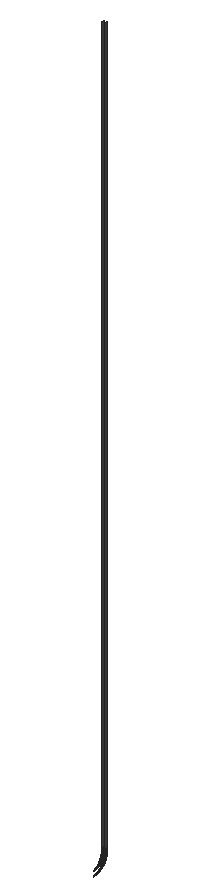
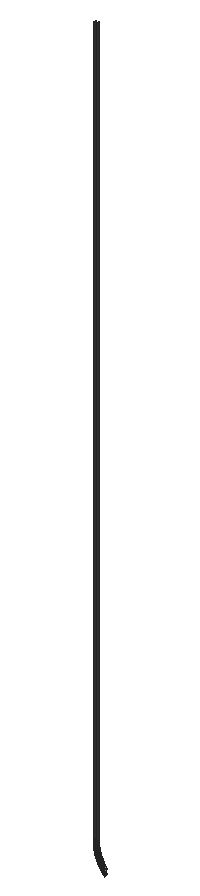
# SketchUp Ruby script. Lengths in inches.
U = 1.inch
M = Sketchup.active_model
def pt(a) = Geom::Point3d.new(a.map { |v| v * U })
def face(e, loops, mat)
  f = e.add_face(loops[0].map { |a| pt(a) })
  loops[1..].each { |l| e.add_face(l.map { |a| pt(a) }).erase! }
  f.material = f.back_material = mat if mat
  f
end
# faces: each face lists its corners as indices into pts; further lists are holes
def faces(e, pts, list, mat = nil) = list.each { |f| face(e, (f[0].is_a?(Array) ? f : [f]).map { |l| l.map { |i| pts[i] } }, mat) }
# xy, xz, yz: faces in a plane at the given z, y or x. An outline is a flat list of corners, or four numbers for a rectangle; further outlines are holes
def ring(l) = l.size == 4 ? [[l[0], l[1]], [l[2], l[1]], [l[2], l[3]], [l[0], l[3]]] : l.each_slice(2).to_a
def flat(e, list, mat, &to3) = list.each { |f| face(e, (f[0].is_a?(Array) ? f : [f]).map { |l| ring(l).map { |u, v| to3.(u, v) } }, mat) }
def xy(e, z, list, mat = nil) = flat(e, list, mat) { |x, y| [x, y, z] }
def xz(e, y, list, mat = nil) = flat(e, list, mat) { |x, z| [x, y, z] }
def yz(e, x, list, mat = nil) = flat(e, list, mat) { |y, z| [x, y, z] }
def lines(e, pts, list) = list.each { |a, b| e.add_line(pt(pts[a]), pt(pts[b])) }
# prism: a flat outline (further loops are holes) pulled along v
def prism(e, loops, v, mat = nil)
  f = face(e, loops, mat); d = Geom::Vector3d.new(v.map { |x| x * U })
  f.pushpull(f.normal.samedirection?(d) ? d.length : -d.length)
end
def box(e, o, s, mat = nil) = prism(e, [[o, [o[0] + s[0], o[1], o[2]], [o[0] + s[0], o[1] + s[1], o[2]], [o[0], o[1] + s[1], o[2]]]], [0, 0, s[2]], mat)
def at(x, y, z, deg = 0) = Geom::Transformation.translation(pt([x, y, z])) * Geom::Transformation.rotation(ORIGIN, Z_AXIS, deg.degrees)
def axes(o, x, y, z) = Geom::Transformation.new([*x, 0, *y, 0, *z, 0, *pt(o).to_a, 1])
def part(name) = M.definitions.add(name)
# library, detail: a bought-in or finely detailed component or shape, given as its bounding box
def library(name, o, s) = part(name).tap { |d| box(d.entities, o, s) }
def detail(e, o, s) = box(e.add_group.entities, o, s)
def put(e, d, t, mat = nil) = e.add_instance(d, t).tap { |i| i.material = mat if mat }
def group(e, t, mat = nil) = e.add_group.tap { |g| g.transformation = t; g.material = mat if mat }.entities
root = M.entities
M.materials.add("1432 AP 8245 TAR ROAD").color = [71, 72, 75]
M.materials.add("Outer Light").color = [251, 217, 152]
yz(root,555.99,[[95.37,191.05,96.87,191.2],[95.37,191.2,96.87,191.34]],"1432 AP 8245 TAR ROAD")
yz(root,555.99,[[95.37,191.05,96.87,191.2],[95.37,191.2,96.87,191.34]],"Outer Light")
yz(root,556,[[95.37,191.49,96.87,191.64],[95.37,191.64,96.87,191.79],[95.37,191.79,96.87,560.79]],"1432 AP 8245 TAR ROAD")
yz(root,556,[[95.37,191.49,96.87,191.64],[95.37,191.64,96.87,191.79],[95.37,191.79,96.87,560.79]],"Outer Light")
yz(root,557.48,[[95.37,190.83,96.87,190.99]],"1432 AP 8245 TAR ROAD")
yz(root,557.48,[[95.37,190.83,96.87,190.99]],"Outer Light")
yz(root,557.49,[[95.37,191.15,96.87,191.31]],"1432 AP 8245 TAR ROAD")
yz(root,557.49,[[95.37,191.15,96.87,191.31]],"Outer Light")
yz(root,557.5,[[95.37,191.47,96.87,191.63],[95.37,191.63,96.87,191.79],[95.37,191.79,96.87,560.79]],"1432 AP 8245 TAR ROAD")
yz(root,557.5,[[95.37,191.47,96.87,191.63],[95.37,191.63,96.87,191.79],[95.37,191.79,96.87,560.79]],"Outer Light")
p = [[551.83,95.37,177.64],[551.94,95.37,177.76],[551.94,96.87,177.76],[551.83,96.87,177.64],[551.83,96.87,177.64],[551.94,96.87,177.76],
  [551.94,95.37,177.76],[551.83,95.37,177.64],[552.05,95.37,177.875],[552.05,96.87,177.875],[552.05,96.87,177.875],[552.05,95.37,177.875],
  [552.16,95.37,178],[552.16,96.87,178],[552.16,96.87,178],[552.16,95.37,178],[552.27,95.37,178.11],[552.27,96.87,178.11],
  [552.27,96.87,178.11],[552.27,95.37,178.11],[552.38,95.37,178.24],[552.38,96.87,178.24],[552.38,96.87,178.24],[552.38,95.37,178.24],
  [552.48,95.37,178.36],[552.48,96.87,178.36],[552.48,96.87,178.36],[552.48,95.37,178.36],[552.59,95.37,178.48],[552.59,96.87,178.48],
  [552.59,96.87,178.48],[552.59,95.37,178.48],[552.69,95.37,178.6],[552.69,96.87,178.6],[552.69,96.87,178.6],[552.69,95.37,178.6],
  [552.8,95.37,178.72],[552.8,96.87,178.72],[552.8,96.87,178.72],[552.8,95.37,178.72],[552.9,95.37,178.85],[552.9,96.87,178.85],
  [552.9,96.87,178.85],[552.9,95.37,178.85],[553,95.37,178.97],[553,96.87,178.97],[553,96.87,178.97],[553,95.37,178.97],
  [553.1,95.37,179.1],[553.1,96.87,179.1],[553.1,96.87,179.1],[553.1,95.37,179.1],[553.2,95.37,179.23],[553.2,96.87,179.23],
  [553.2,96.87,179.23],[553.2,95.37,179.23],[553.3,95.37,179.36],[553.3,96.87,179.36],[553.3,96.87,179.36],[553.3,95.37,179.36],
  [553.39,95.37,179.48],[553.39,96.87,179.48],[553.39,96.87,179.48],[553.39,95.37,179.48],[553.49,95.37,179.61],[553.49,96.87,179.61],
  [553.49,96.87,179.61],[553.49,95.37,179.61],[553.58,95.37,179.74],[553.58,96.87,179.74],[553.58,96.87,179.74],[553.58,95.37,179.74],
  [553.68,95.37,179.875],[553.68,96.87,179.875],[553.68,96.87,179.875],[553.68,95.37,179.875],[551.92,95.37,180.03],[551.83,95.37,179.91],
  [551.83,96.87,179.91],[551.92,96.87,180.03],[551.92,96.87,180.03],[551.83,96.87,179.91],[551.83,95.37,179.91],[551.92,95.37,180.03],
  [553.77,95.37,180],[553.77,96.87,180],[553.77,96.87,180],[553.77,95.37,180],[552.01,95.37,180.15],[552.01,96.87,180.15],
  [552.01,96.87,180.15],[552.01,95.37,180.15],[553.86,95.37,180.14],[553.86,96.87,180.14],[553.86,96.87,180.14],[553.86,95.37,180.14],
  [552.1,95.37,180.27],[552.1,96.87,180.27],[552.1,96.87,180.27],[552.1,95.37,180.27],[553.96,95.37,180.27],[553.96,96.87,180.27],
  [553.96,96.87,180.27],[553.96,95.37,180.27],[552.19,95.37,180.38],[552.19,96.87,180.38],[552.19,96.87,180.38],[552.19,95.37,180.38],
  [554.05,95.37,180.4],[554.05,96.87,180.4],[554.05,96.87,180.4],[554.05,95.37,180.4],[552.28,95.37,180.5],[552.28,96.87,180.5],
  [552.28,96.87,180.5],[552.28,95.37,180.5],[554.13,95.37,180.54],[554.13,96.87,180.54],[554.13,96.87,180.54],[554.13,95.37,180.54],
  [552.37,95.37,180.625],[552.37,96.87,180.625],[552.37,96.87,180.625],[552.37,95.37,180.625],[554.22,95.37,180.67],[554.22,96.87,180.67],
  [554.22,96.87,180.67],[554.22,95.37,180.67],[552.46,95.37,180.75],[552.46,96.87,180.75],[552.46,96.87,180.75],[552.46,95.37,180.75],
  [552.54,95.37,180.87],[552.54,96.87,180.87],[552.54,96.87,180.87],[552.54,95.37,180.87],[554.31,95.37,180.81],[554.31,96.87,180.81],
  [554.31,96.87,180.81],[554.31,95.37,180.81],[554.39,95.37,180.94],[554.39,96.87,180.94],[554.39,96.87,180.94],[554.39,95.37,180.94],
  [552.63,95.37,180.99],[552.63,96.87,180.99],[552.63,96.87,180.99],[552.63,95.37,180.99],[554.48,95.37,181.08],[554.48,96.87,181.08],
  [554.48,96.87,181.08],[554.48,95.37,181.08],[552.71,95.37,181.11],[552.71,96.87,181.11],[552.71,96.87,181.11],[552.71,95.37,181.11],
  [552.8,95.37,181.24],[552.8,96.87,181.24],[552.8,96.87,181.24],[552.8,95.37,181.24],[554.5625,95.37,181.22],[554.5625,96.87,181.22],
  [554.5625,96.87,181.22],[554.5625,95.37,181.22],[552.88,95.37,181.36],[552.88,96.87,181.36],[552.88,96.87,181.36],[552.88,95.37,181.36],
  [554.65,95.37,181.36],[554.65,96.87,181.36],[554.65,96.87,181.36],[554.65,95.37,181.36],[552.96,95.37,181.49],[552.96,96.87,181.49],
  [552.96,96.87,181.49],[552.96,95.37,181.49],[554.73,95.37,181.5],[554.73,96.87,181.5],[554.73,96.87,181.5],[554.73,95.37,181.5],
  [553.04,95.37,181.61],[553.04,96.87,181.61],[553.04,96.87,181.61],[553.04,95.37,181.61],[554.81,95.37,181.64],[554.81,96.87,181.64],
  [554.81,96.87,181.64],[554.81,95.37,181.64],[553.12,95.37,181.74],[553.12,96.87,181.74],[553.12,96.87,181.74],[553.12,95.37,181.74],
  [554.89,95.37,181.78],[554.89,96.87,181.78],[554.89,96.87,181.78],[554.89,95.37,181.78],[553.2,95.37,181.86],[553.2,96.87,181.86],
  [553.2,96.87,181.86],[553.2,95.37,181.86],[554.96,95.37,181.92],[554.96,96.87,181.92],[554.96,96.87,181.92],[554.96,95.37,181.92],
  [553.28,95.37,181.99],[553.28,96.87,181.99],[553.28,96.87,181.99],[553.28,95.37,181.99],[555.04,95.37,182.06],[555.04,96.87,182.06],
  [555.04,96.87,182.06],[555.04,95.37,182.06],[553.35,95.37,182.12],[553.35,96.87,182.12],[553.35,96.87,182.12],[553.35,95.37,182.12],
  [553.43,95.37,182.25],[553.43,96.87,182.25],[553.43,96.87,182.25],[553.43,95.37,182.25],[555.12,95.37,182.2],[555.12,96.87,182.2],
  [555.12,96.87,182.2],[555.12,95.37,182.2],[553.5,95.37,182.38],[553.5,96.87,182.38],[553.5,96.87,182.38],[553.5,95.37,182.38],
  [555.19,95.37,182.34],[555.19,96.87,182.34],[555.19,96.87,182.34],[555.19,95.37,182.34],[555.27,95.37,182.49],[555.27,96.87,182.49],
  [555.27,96.87,182.49],[555.27,95.37,182.49],[553.58,95.37,182.51],[553.58,96.87,182.51],[553.58,96.87,182.51],[553.58,95.37,182.51],
  [553.65,95.37,182.64],[553.65,96.87,182.64],[553.65,96.87,182.64],[553.65,95.37,182.64],[555.34,95.37,182.63],[555.34,96.87,182.63],
  [555.34,96.87,182.63],[555.34,95.37,182.63],[553.72,95.37,182.77],[553.72,96.87,182.77],[553.72,96.87,182.77],[553.72,95.37,182.77],
  [555.41,95.37,182.77],[555.41,96.87,182.77],[555.41,96.87,182.77],[555.41,95.37,182.77],[553.79,95.37,182.9],[553.79,96.87,182.9],
  [553.79,96.87,182.9],[553.79,95.37,182.9],[555.48,95.37,182.92],[555.48,96.87,182.92],[555.48,96.87,182.92],[555.48,95.37,182.92],
  [553.86,95.37,183.03],[553.86,96.87,183.03],[553.86,96.87,183.03],[553.86,95.37,183.03],[555.55,95.37,183.0625],[555.55,96.87,183.0625],
  [555.55,96.87,183.0625],[555.55,95.37,183.0625],[553.93,95.37,183.17],[553.93,96.87,183.17],[553.93,96.87,183.17],[553.93,95.37,183.17],
  [555.62,95.37,183.21],[555.62,96.87,183.21],[555.62,96.87,183.21],[555.62,95.37,183.21],[554,95.37,183.3],[554,96.87,183.3],
  [554,96.87,183.3],[554,95.37,183.3],[555.68,95.37,183.36],[555.68,96.87,183.36],[555.68,96.87,183.36],[555.68,95.37,183.36],
  [554.0625,95.37,183.43],[554.0625,96.87,183.43],[554.0625,96.87,183.43],[554.0625,95.37,183.43],[554.13,95.37,183.57],[554.13,96.87,183.57],
  [554.13,96.87,183.57],[554.13,95.37,183.57],[555.75,95.37,183.5],[555.75,96.87,183.5],[555.75,96.87,183.5],[555.75,95.37,183.5],
  [555.8125,95.37,183.65],[555.8125,96.87,183.65],[555.8125,96.87,183.65],[555.8125,95.37,183.65],[554.19,95.37,183.7],[554.19,96.87,183.7],
  [554.19,96.87,183.7],[554.19,95.37,183.7],[554.25,95.37,183.84],[554.25,96.87,183.84],[554.25,96.87,183.84],[554.25,95.37,183.84],
  [555.88,95.37,183.8],[555.88,96.87,183.8],[555.88,96.87,183.8],[555.88,95.37,183.8],[554.32,95.37,183.97],[554.32,96.87,183.97],
  [554.32,96.87,183.97],[554.32,95.37,183.97],[555.94,95.37,183.95],[555.94,96.87,183.95],[555.94,96.87,183.95],[555.94,95.37,183.95],
  [556,95.37,184.1],[556,96.87,184.1],[556,96.87,184.1],[556,95.37,184.1],[554.38,95.37,184.11],[554.38,96.87,184.11],
  [554.38,96.87,184.11],[554.38,95.37,184.11],[554.4375,95.37,184.25],[554.4375,96.87,184.25],[554.4375,96.87,184.25],[554.4375,95.37,184.25],
  [556.06,95.37,184.25],[556.06,96.87,184.25],[556.06,96.87,184.25],[556.06,95.37,184.25],[554.5,95.37,184.38],[554.5,96.87,184.38],
  [554.5,96.87,184.38],[554.5,95.37,184.38],[556.12,95.37,184.4],[556.12,96.87,184.4],[556.12,96.87,184.4],[556.12,95.37,184.4],
  [554.55,95.37,184.52],[554.55,96.87,184.52],[554.55,96.87,184.52],[554.55,95.37,184.52],[556.18,95.37,184.55],[556.18,96.87,184.55],
  [556.18,96.87,184.55],[556.18,95.37,184.55],[554.61,95.37,184.66],[554.61,96.87,184.66],[554.61,96.87,184.66],[554.61,95.37,184.66],
  [556.23,95.37,184.7],[556.23,96.87,184.7],[556.23,96.87,184.7],[556.23,95.37,184.7],[554.67,95.37,184.8],[554.67,96.87,184.8],
  [554.67,96.87,184.8],[554.67,95.37,184.8],[556.29,95.37,184.85],[556.29,96.87,184.85],[556.29,96.87,184.85],[556.29,95.37,184.85],
  [554.72,95.37,184.9375],[554.72,96.87,184.9375],[554.72,96.87,184.9375],[554.72,95.37,184.9375],[556.34,95.37,185],[556.34,96.87,185],
  [556.34,96.87,185],[556.34,95.37,185],[554.77,95.37,185.08],[554.77,96.87,185.08],[554.77,96.87,185.08],[554.77,95.37,185.08],
  [556.39,95.37,185.15],[556.39,96.87,185.15],[556.39,96.87,185.15],[556.39,95.37,185.15],[554.83,95.37,185.22],[554.83,96.87,185.22],
  [554.83,96.87,185.22],[554.83,95.37,185.22],[554.875,95.37,185.36],[554.875,96.87,185.36],[554.875,96.87,185.36],[554.875,95.37,185.36],
  [556.45,95.37,185.3],[556.45,96.87,185.3],[556.45,96.87,185.3],[556.45,95.37,185.3],[556.5,95.37,185.46],[556.5,96.87,185.46],
  [556.5,96.87,185.46],[556.5,95.37,185.46],[554.93,95.37,185.5],[554.93,96.87,185.5],[554.93,96.87,185.5],[554.93,95.37,185.5],
  [554.98,95.37,185.64],[554.98,96.87,185.64],[554.98,96.87,185.64],[554.98,95.37,185.64],[556.55,95.37,185.61],[556.55,96.87,185.61],
  [556.55,96.87,185.61],[556.55,95.37,185.61],[555.02,95.37,185.78],[555.02,96.87,185.78],[555.02,96.87,185.78],[555.02,95.37,185.78],
  [556.59,95.37,185.76],[556.59,96.87,185.76],[556.59,96.87,185.76],[556.59,95.37,185.76],[555.07,95.37,185.92],[555.07,96.87,185.92],
  [555.07,96.87,185.92],[555.07,95.37,185.92],[556.64,95.37,185.92],[556.64,96.87,185.92],[556.64,96.87,185.92],[556.64,95.37,185.92],
  [555.12,95.37,186.0625],[555.12,96.87,186.0625],[555.12,96.87,186.0625],[555.12,95.37,186.0625],[556.6875,95.37,186.07],[556.6875,96.87,186.07],
  [556.6875,96.87,186.07],[556.6875,95.37,186.07],[555.16,95.37,186.21],[555.16,96.87,186.21],[555.16,96.87,186.21],[555.16,95.37,186.21],
  [556.73,95.37,186.23],[556.73,96.87,186.23],[556.73,96.87,186.23],[556.73,95.37,186.23],[555.2,95.37,186.35],[555.2,96.87,186.35],
  [555.2,96.87,186.35],[555.2,95.37,186.35],[556.77,95.37,186.38],[556.77,96.87,186.38],[556.77,96.87,186.38],[556.77,95.37,186.38],
  [555.25,95.37,186.49],[555.25,96.87,186.49],[555.25,96.87,186.49],[555.25,95.37,186.49],[556.82,95.37,186.54],[556.82,96.87,186.54],
  [556.82,96.87,186.54],[556.82,95.37,186.54],[555.29,95.37,186.63],[555.29,96.87,186.63],[555.29,96.87,186.63],[555.29,95.37,186.63],
  [556.86,95.37,186.69],[556.86,96.87,186.69],[556.86,96.87,186.69],[556.86,95.37,186.69],[555.33,95.37,186.78],[555.33,96.87,186.78],
  [555.33,96.87,186.78],[555.33,95.37,186.78],[556.9,95.37,186.85],[556.9,96.87,186.85],[556.9,96.87,186.85],[556.9,95.37,186.85],
  [555.37,95.37,186.92],[555.37,96.87,186.92],[555.37,96.87,186.92],[555.37,95.37,186.92],[555.4,95.37,187.07],[555.4,96.87,187.07],
  [555.4,96.87,187.07],[555.4,95.37,187.07],[556.93,95.37,187.01],[556.93,96.87,187.01],[556.93,96.87,187.01],[556.93,95.37,187.01],
  [556.97,95.37,187.16],[556.97,96.87,187.16],[556.97,96.87,187.16],[556.97,95.37,187.16],[555.44,95.37,187.21],[555.44,96.87,187.21],
  [555.44,96.87,187.21],[555.44,95.37,187.21],[555.48,95.37,187.36],[555.48,96.87,187.36],[555.48,96.87,187.36],[555.48,95.37,187.36],
  [557.01,95.37,187.32],[557.01,96.87,187.32],[557.01,96.87,187.32],[557.01,95.37,187.32],[557.04,95.37,187.48],[557.04,96.87,187.48],
  [557.04,96.87,187.48],[557.04,95.37,187.48],[555.51,95.37,187.5],[555.51,96.87,187.5],[555.51,96.87,187.5],[555.51,95.37,187.5],
  [555.54,95.37,187.65],[555.54,96.87,187.65],[555.54,96.87,187.65],[555.54,95.37,187.65],[557.07,95.37,187.63],[557.07,96.87,187.63],
  [557.07,96.87,187.63],[557.07,95.37,187.63],[555.57,95.37,187.79],[555.57,96.87,187.79],[555.57,96.87,187.79],[555.57,95.37,187.79],
  [557.11,95.37,187.79],[557.11,96.87,187.79],[557.11,96.87,187.79],[557.11,95.37,187.79],[555.61,95.37,187.9375],[555.61,96.87,187.9375],
  [555.61,96.87,187.9375],[555.61,95.37,187.9375],[557.14,95.37,187.95],[557.14,96.87,187.95],[557.14,96.87,187.95],[557.14,95.37,187.95],
  [555.63,95.37,188.09],[555.63,96.87,188.09],[555.63,96.87,188.09],[555.63,95.37,188.09],[557.17,95.37,188.11],[557.17,96.87,188.11],
  [557.17,96.87,188.11],[557.17,95.37,188.11],[555.66,95.37,188.23],[555.66,96.87,188.23],[555.66,96.87,188.23],[555.66,95.37,188.23],
  [557.19,95.37,188.27],[557.19,96.87,188.27],[557.19,96.87,188.27],[557.19,95.37,188.27],[555.69,95.37,188.38],[555.69,96.87,188.38],
  [555.69,96.87,188.38],[555.69,95.37,188.38],[557.22,95.37,188.43],[557.22,96.87,188.43],[557.22,96.87,188.43],[557.22,95.37,188.43],
  [555.72,95.37,188.53],[555.72,96.87,188.53],[555.72,96.87,188.53],[555.72,95.37,188.53],[557.25,95.37,188.59],[557.25,96.87,188.59],
  [557.25,96.87,188.59],[557.25,95.37,188.59],[555.74,95.37,188.67],[555.74,96.87,188.67],[555.74,96.87,188.67],[555.74,95.37,188.67],
  [557.27,95.37,188.74],[557.27,96.87,188.74],[557.27,96.87,188.74],[557.27,95.37,188.74],[555.77,95.37,188.82],[555.77,96.87,188.82],
  [555.77,96.87,188.82],[555.77,95.37,188.82],[557.3,95.37,188.9],[557.3,96.87,188.9],[557.3,96.87,188.9],[557.3,95.37,188.9],
  [555.79,95.37,188.97],[555.79,96.87,188.97],[555.79,96.87,188.97],[555.79,95.37,188.97],[557.32,95.37,189.0625],[557.32,96.87,189.0625],
  [557.32,96.87,189.0625],[557.32,95.37,189.0625],[555.81,95.37,189.11],[555.81,96.87,189.11],[555.81,96.87,189.11],[555.81,95.37,189.11],
  [555.83,95.37,189.26],[555.83,96.87,189.26],[555.83,96.87,189.26],[555.83,95.37,189.26],[557.34,95.37,189.22],[557.34,96.87,189.22],
  [557.34,96.87,189.22],[557.34,95.37,189.22],[557.36,95.37,189.38],[557.36,96.87,189.38],[557.36,96.87,189.38],[557.36,95.37,189.38],
  [555.85,95.37,189.41],[555.85,96.87,189.41],[555.85,96.87,189.41],[555.85,95.37,189.41],[555.87,95.37,189.56],[555.87,96.87,189.56],
  [555.87,96.87,189.56],[555.87,95.37,189.56],[557.375,95.37,189.54],[557.375,96.87,189.54],[557.375,96.87,189.54],[557.375,95.37,189.54],
  [557.39,95.37,189.7],[557.39,96.87,189.7],[557.39,96.87,189.7],[557.39,95.37,189.7],[555.89,95.37,189.71],[555.89,96.87,189.71],
  [555.89,96.87,189.71],[555.89,95.37,189.71],[555.9,95.37,189.86],[555.9,96.87,189.86],[555.9,96.87,189.86],[555.9,95.37,189.86],
  [557.41,95.37,189.86],[557.41,96.87,189.86],[557.41,96.87,189.86],[557.41,95.37,189.86],[555.92,95.37,190],[555.92,96.87,190],
  [555.92,96.87,190],[555.92,95.37,190],[557.42,95.37,190.02],[557.42,96.87,190.02],[557.42,96.87,190.02],[557.42,95.37,190.02],
  [555.93,95.37,190.15],[555.93,96.87,190.15],[555.93,96.87,190.15],[555.93,95.37,190.15],[557.4375,95.37,190.18],[557.4375,96.87,190.18],
  [557.4375,96.87,190.18],[557.4375,95.37,190.18],[555.94,95.37,190.3],[555.94,96.87,190.3],[555.94,96.87,190.3],[555.94,95.37,190.3],
  [557.45,95.37,190.34],[557.45,96.87,190.34],[557.45,96.87,190.34],[557.45,95.37,190.34],[555.95,95.37,190.45],[555.95,96.87,190.45],
  [555.95,96.87,190.45],[555.95,95.37,190.45],[557.46,95.37,190.5],[557.46,96.87,190.5],[557.46,96.87,190.5],[557.46,95.37,190.5],
  [555.96,95.37,190.6],[555.96,96.87,190.6],[555.96,96.87,190.6],[555.96,95.37,190.6],[557.47,95.37,190.67],[557.47,96.87,190.67],
  [557.47,96.87,190.67],[557.47,95.37,190.67],[555.97,95.37,190.75],[555.97,96.87,190.75],[555.97,96.87,190.75],[555.97,95.37,190.75],
  [555.98,95.37,190.9],[555.98,96.87,190.9],[555.98,96.87,190.9],[555.98,95.37,190.9],[557.48,95.37,190.83],[557.48,96.87,190.83],
  [557.48,96.87,190.83],[557.48,95.37,190.83],[555.99,95.37,191.05],[555.99,96.87,191.05],[555.99,96.87,191.05],[555.99,95.37,191.05],
  [557.48,95.37,190.99],[557.49,95.37,191.15],[557.49,96.87,191.15],[557.48,96.87,190.99],[557.48,96.87,190.99],[557.49,96.87,191.15],
  [557.49,95.37,191.15],[557.48,95.37,190.99],[556,95.37,191.49],[555.99,95.37,191.34],[555.99,96.87,191.34],[556,96.87,191.49],
  [556,96.87,191.49],[555.99,96.87,191.34],[555.99,95.37,191.34],[556,95.37,191.49],[557.49,95.37,191.31],[557.5,95.37,191.47],
  [557.5,96.87,191.47],[557.49,96.87,191.31],[557.49,96.87,191.31],[557.5,96.87,191.47],[557.5,95.37,191.47],[557.49,95.37,191.31]]
faces(root,p,[[0,1,2,3],[1,8,9,2],[8,12,13,9],[12,16,17,13],[16,20,21,17],[20,24,25,21],[24,28,29,25],[28,32,33,29],
  [32,36,37,33],[36,40,41,37],[40,44,45,41],[44,48,49,45],[48,52,53,49],[52,56,57,53],[56,60,61,57],[60,64,65,61],
  [64,68,69,65],[68,72,73,69],[76,77,78,79],[72,84,85,73],[88,76,79,89],[84,92,93,85],[96,88,89,97],[92,100,101,93],
  [104,96,97,105],[100,108,109,101],[112,104,105,113],[108,116,117,109],[120,112,113,121],[116,124,125,117],[128,120,121,129],[132,128,129,133],
  [124,136,137,125],[136,140,141,137],[144,132,133,145],[140,148,149,141],[152,144,145,153],[156,152,153,157],[148,160,161,149],[164,156,157,165],
  [160,168,169,161],[172,164,165,173],[168,176,177,169],[180,172,173,181],[176,184,185,177],[188,180,181,189],[184,192,193,185],[196,188,189,197],
  [192,200,201,193],[204,196,197,205],[200,208,209,201],[212,204,205,213],[216,212,213,217],[208,220,221,209],[224,216,217,225],[220,228,229,221],
  [228,232,233,229],[236,224,225,237],[240,236,237,241],[232,244,245,233],[248,240,241,249],[244,252,253,245],[256,248,249,257],[252,260,261,253],
  [264,256,257,265],[260,268,269,261],[272,264,265,273],[268,276,277,269],[280,272,273,281],[276,284,285,277],[288,280,281,289],[292,288,289,293],
  [284,296,297,285],[296,300,301,297],[304,292,293,305],[308,304,305,309],[300,312,313,301],[316,308,309,317],[312,320,321,313],[320,324,325,321],
  [328,316,317,329],[332,328,329,333],[324,336,337,325],[340,332,333,341],[336,344,345,337],[348,340,341,349],[344,352,353,345],[356,348,349,357],
  [352,360,361,353],[364,356,357,365],[360,368,369,361],[372,364,365,373],[368,376,377,369],[380,372,373,381],[376,384,385,377],[388,380,381,389],
  [392,388,389,393],[384,396,397,385],[396,400,401,397],[404,392,393,405],[408,404,405,409],[400,412,413,401],[416,408,409,417],[412,420,421,413],
  [424,416,417,425],[420,428,429,421],[432,424,425,433],[428,436,437,429],[440,432,433,441],[436,444,445,437],[448,440,441,449],[444,452,453,445],
  [456,448,449,457],[452,460,461,453],[464,456,457,465],[460,468,469,461],[472,464,465,473],[468,476,477,469],[480,472,473,481],[484,480,481,485],
  [476,488,489,477],[488,492,493,489],[496,484,485,497],[500,496,497,501],[492,504,505,493],[504,508,509,505],[512,500,501,513],[516,512,513,517],
  [508,520,521,509],[524,516,517,525],[520,528,529,521],[532,524,525,533],[528,536,537,529],[540,532,533,541],[536,544,545,537],[548,540,541,549],
  [544,552,553,545],[556,548,549,557],[552,560,561,553],[564,556,557,565],[560,568,569,561],[572,564,565,573],[568,576,577,569],[580,572,573,581],
  [576,584,585,577],[588,580,581,589],[584,592,593,585],[596,588,589,597],[600,596,597,601],[592,604,605,593],[604,608,609,605],[612,600,601,613],
  [616,612,613,617],[608,620,621,609],[620,624,625,621],[628,616,617,629],[632,628,629,633],[624,636,637,625],[640,632,633,641],[636,644,645,637],
  [648,640,641,649],[644,652,653,645],[656,648,649,657],[652,660,661,653],[664,656,657,665],[660,668,669,661],[672,664,665,673],[668,676,677,669],
  [680,672,673,681],[684,680,681,685],[676,688,689,677],[692,684,685,693],[696,697,698,699],[704,705,706,707],[712,713,714,715]],"1432 AP 8245 TAR ROAD")
faces(root,p,[[4,5,6,7],[5,10,11,6],[10,14,15,11],[14,18,19,15],[18,22,23,19],[22,26,27,23],[26,30,31,27],[30,34,35,31],
  [34,38,39,35],[38,42,43,39],[42,46,47,43],[46,50,51,47],[50,54,55,51],[54,58,59,55],[58,62,63,59],[62,66,67,63],
  [66,70,71,67],[70,74,75,71],[80,81,82,83],[74,86,87,75],[90,80,83,91],[86,94,95,87],[98,90,91,99],[94,102,103,95],
  [106,98,99,107],[102,110,111,103],[114,106,107,115],[110,118,119,111],[122,114,115,123],[118,126,127,119],[130,122,123,131],[134,130,131,135],
  [126,138,139,127],[138,142,143,139],[146,134,135,147],[142,150,151,143],[154,146,147,155],[158,154,155,159],[150,162,163,151],[166,158,159,167],
  [162,170,171,163],[174,166,167,175],[170,178,179,171],[182,174,175,183],[178,186,187,179],[190,182,183,191],[186,194,195,187],[198,190,191,199],
  [194,202,203,195],[206,198,199,207],[202,210,211,203],[214,206,207,215],[218,214,215,219],[210,222,223,211],[226,218,219,227],[222,230,231,223],
  [230,234,235,231],[238,226,227,239],[242,238,239,243],[234,246,247,235],[250,242,243,251],[246,254,255,247],[258,250,251,259],[254,262,263,255],
  [266,258,259,267],[262,270,271,263],[274,266,267,275],[270,278,279,271],[282,274,275,283],[278,286,287,279],[290,282,283,291],[294,290,291,295],
  [286,298,299,287],[298,302,303,299],[306,294,295,307],[310,306,307,311],[302,314,315,303],[318,310,311,319],[314,322,323,315],[322,326,327,323],
  [330,318,319,331],[334,330,331,335],[326,338,339,327],[342,334,335,343],[338,346,347,339],[350,342,343,351],[346,354,355,347],[358,350,351,359],
  [354,362,363,355],[366,358,359,367],[362,370,371,363],[374,366,367,375],[370,378,379,371],[382,374,375,383],[378,386,387,379],[390,382,383,391],
  [394,390,391,395],[386,398,399,387],[398,402,403,399],[406,394,395,407],[410,406,407,411],[402,414,415,403],[418,410,411,419],[414,422,423,415],
  [426,418,419,427],[422,430,431,423],[434,426,427,435],[430,438,439,431],[442,434,435,443],[438,446,447,439],[450,442,443,451],[446,454,455,447],
  [458,450,451,459],[454,462,463,455],[466,458,459,467],[462,470,471,463],[474,466,467,475],[470,478,479,471],[482,474,475,483],[486,482,483,487],
  [478,490,491,479],[490,494,495,491],[498,486,487,499],[502,498,499,503],[494,506,507,495],[506,510,511,507],[514,502,503,515],[518,514,515,519],
  [510,522,523,511],[526,518,519,527],[522,530,531,523],[534,526,527,535],[530,538,539,531],[542,534,535,543],[538,546,547,539],[550,542,543,551],
  [546,554,555,547],[558,550,551,559],[554,562,563,555],[566,558,559,567],[562,570,571,563],[574,566,567,575],[570,578,579,571],[582,574,575,583],
  [578,586,587,579],[590,582,583,591],[586,594,595,587],[598,590,591,599],[602,598,599,603],[594,606,607,595],[606,610,611,607],[614,602,603,615],
  [618,614,615,619],[610,622,623,611],[622,626,627,623],[630,618,619,631],[634,630,631,635],[626,638,639,627],[642,634,635,643],[638,646,647,639],
  [650,642,643,651],[646,654,655,647],[658,650,651,659],[654,662,663,655],[666,658,659,667],[662,670,671,663],[674,666,667,675],[670,678,679,671],
  [682,674,675,683],[686,682,683,687],[678,690,691,679],[694,686,687,695],[700,701,702,703],[708,709,710,711],[716,717,718,719]],"Outer Light")
